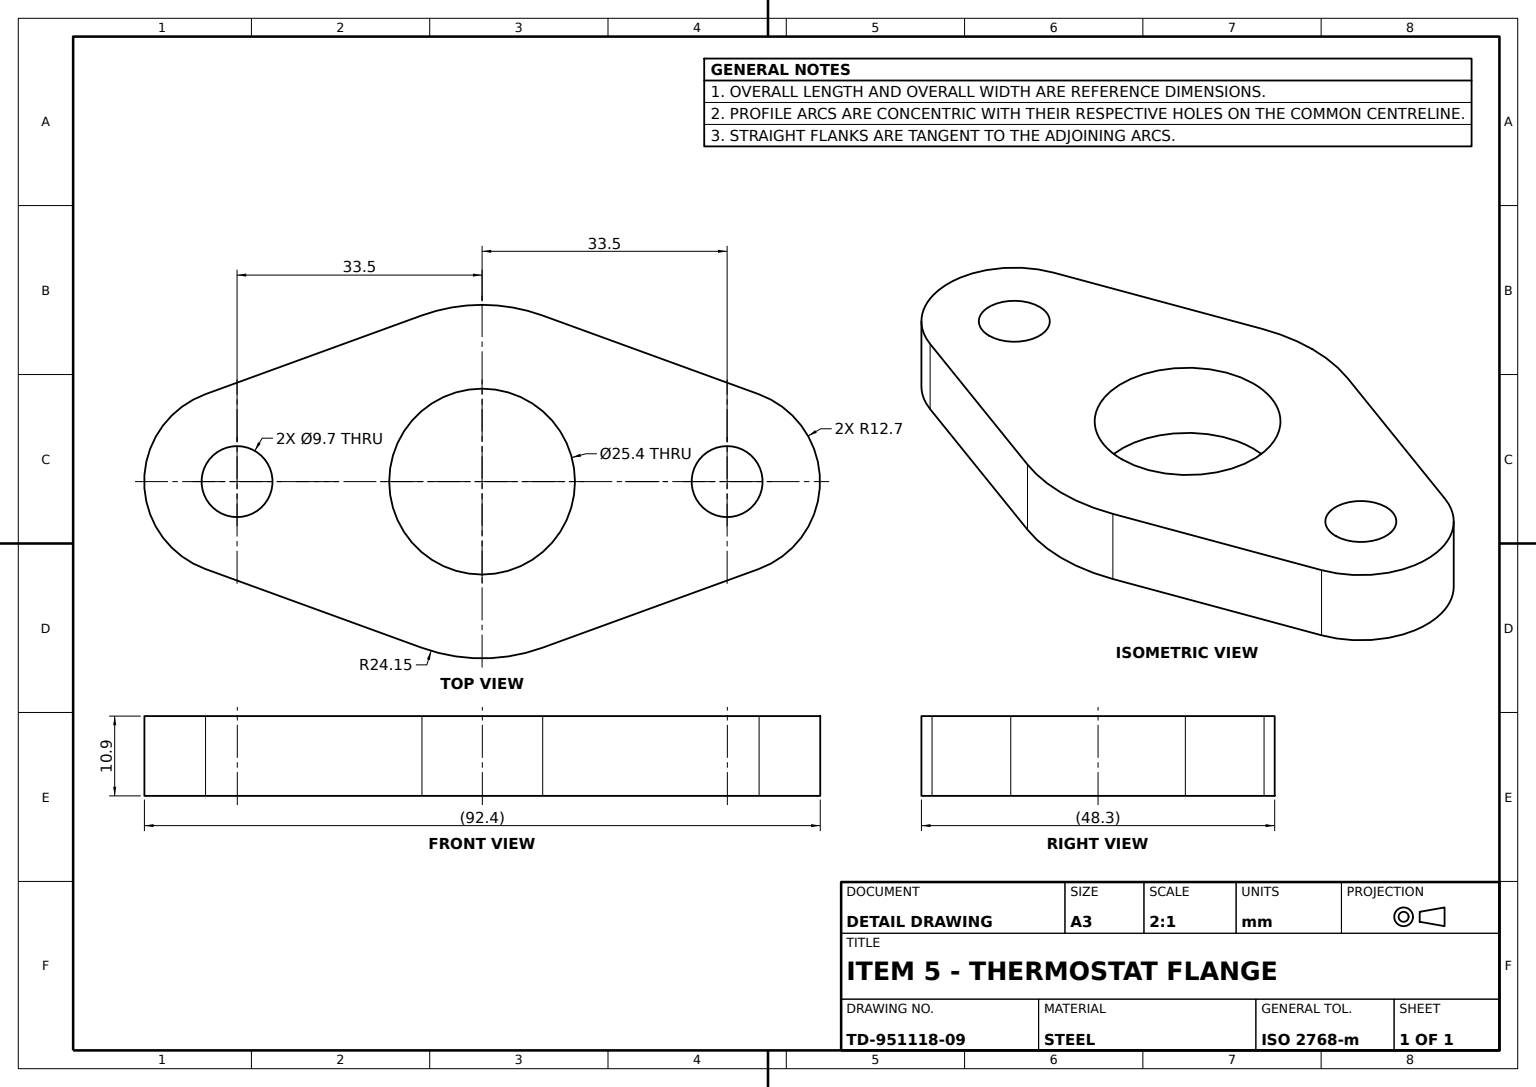
ISO-10303-21;
HEADER;
FILE_DESCRIPTION((''),'2;1');
FILE_NAME('','',(''),(''),'','','');
FILE_SCHEMA(('AUTOMOTIVE_DESIGN'));
ENDSEC;
DATA;
#1=APPLICATION_CONTEXT('');
#2=PRODUCT_CONTEXT('',#1,'mechanical');
#3=PRODUCT('','','',(#2));
#4=PRODUCT_DEFINITION_FORMATION('','',#3);
#5=PRODUCT_DEFINITION_CONTEXT('',#1,'design');
#6=PRODUCT_DEFINITION('','',#4,#5);
#7=PRODUCT_DEFINITION_SHAPE('','',#6);
#8=(LENGTH_UNIT()NAMED_UNIT(*)SI_UNIT(.MILLI.,.METRE.));
#9=(NAMED_UNIT(*)PLANE_ANGLE_UNIT()SI_UNIT($,.RADIAN.));
#10=(NAMED_UNIT(*)SI_UNIT($,.STERADIAN.)SOLID_ANGLE_UNIT());
#11=UNCERTAINTY_MEASURE_WITH_UNIT(LENGTH_MEASURE(1.E-05),#8,'distance_accuracy_value','');
#12=(GEOMETRIC_REPRESENTATION_CONTEXT(3)GLOBAL_UNCERTAINTY_ASSIGNED_CONTEXT((#11))GLOBAL_UNIT_ASSIGNED_CONTEXT((#8,#9,#10))REPRESENTATION_CONTEXT('',''));
#13=CARTESIAN_POINT('',(-12.7,0.,10.9));
#14=VERTEX_POINT('',#13);
#15=CARTESIAN_POINT('',(12.7,0.,10.9));
#16=VERTEX_POINT('',#15);
#17=CARTESIAN_POINT('',(0.,0.,10.9));
#18=DIRECTION('',(0.,0.,1.));
#19=DIRECTION('',(1.,0.,0.));
#20=AXIS2_PLACEMENT_3D('',#17,#18,#19);
#21=CIRCLE('',#20,12.7);
#22=EDGE_CURVE('',#14,#16,#21,.T.);
#23=ORIENTED_EDGE('',*,*,#22,.T.);
#24=CARTESIAN_POINT('',(12.7,0.,0.));
#25=VERTEX_POINT('',#24);
#26=CARTESIAN_POINT('',(12.7,0.,-39.));
#27=VECTOR('',#18,1000.);
#28=LINE('',#26,#27);
#29=EDGE_CURVE('',#25,#16,#28,.T.);
#30=ORIENTED_EDGE('',*,*,#29,.F.);
#31=CARTESIAN_POINT('',(-12.7,0.,0.));
#32=VERTEX_POINT('',#31);
#33=CARTESIAN_POINT('',(0.,0.,0.));
#34=DIRECTION('',(0.,0.,-1.));
#35=DIRECTION('',(-1.,0.,0.));
#36=AXIS2_PLACEMENT_3D('',#33,#34,#35);
#37=CIRCLE('',#36,12.7);
#38=EDGE_CURVE('',#25,#32,#37,.T.);
#39=ORIENTED_EDGE('',*,*,#38,.T.);
#40=CARTESIAN_POINT('',(-12.7,0.,-39.));
#41=LINE('',#40,#27);
#42=EDGE_CURVE('',#32,#14,#41,.T.);
#43=ORIENTED_EDGE('',*,*,#42,.T.);
#44=EDGE_LOOP('',(#23,#30,#39,#43));
#45=FACE_OUTER_BOUND('',#44,.T.);
#46=CARTESIAN_POINT('',(0.,0.,-39.));
#47=AXIS2_PLACEMENT_3D('',#46,#18,#19);
#48=CYLINDRICAL_SURFACE('',#47,12.7);
#49=ADVANCED_FACE('',(#45),#48,.F.);
#50=CARTESIAN_POINT('',(22.69559,8.254254,10.9));
#51=VERTEX_POINT('',#50);
#52=CARTESIAN_POINT('',(11.935155,37.840746,10.9));
#53=VERTEX_POINT('',#52);
#54=DIRECTION('',(-0.341791045,0.939775974,0.));
#55=VECTOR('',#54,1000.);
#56=LINE('',#52,#55);
#57=EDGE_CURVE('',#51,#53,#56,.T.);
#58=ORIENTED_EDGE('',*,*,#57,.T.);
#59=CARTESIAN_POINT('',(-11.935155,37.840746,10.9));
#60=VERTEX_POINT('',#59);
#61=CARTESIAN_POINT('',(0.,33.5,10.9));
#62=AXIS2_PLACEMENT_3D('',#61,#18,#19);
#63=CIRCLE('',#62,12.7);
#64=EDGE_CURVE('',#53,#60,#63,.T.);
#65=ORIENTED_EDGE('',*,*,#64,.T.);
#66=CARTESIAN_POINT('',(-22.69559,8.254254,10.9));
#67=VERTEX_POINT('',#66);
#68=DIRECTION('',(-0.341791045,-0.939775974,0.));
#69=VECTOR('',#68,1000.);
#70=LINE('',#59,#69);
#71=EDGE_CURVE('',#60,#67,#70,.T.);
#72=ORIENTED_EDGE('',*,*,#71,.T.);
#73=CARTESIAN_POINT('',(-24.15,0.,10.9));
#74=VERTEX_POINT('',#73);
#75=CIRCLE('',#20,24.15);
#76=EDGE_CURVE('',#67,#74,#75,.T.);
#77=ORIENTED_EDGE('',*,*,#76,.T.);
#78=CARTESIAN_POINT('',(-22.69559,-8.254254,10.9));
#79=VERTEX_POINT('',#78);
#80=EDGE_CURVE('',#74,#79,#75,.T.);
#81=ORIENTED_EDGE('',*,*,#80,.T.);
#82=CARTESIAN_POINT('',(-11.935155,-37.840746,10.9));
#83=VERTEX_POINT('',#82);
#84=DIRECTION('',(0.341791045,-0.939775974,0.));
#85=VECTOR('',#84,1000.);
#86=LINE('',#82,#85);
#87=EDGE_CURVE('',#79,#83,#86,.T.);
#88=ORIENTED_EDGE('',*,*,#87,.T.);
#89=CARTESIAN_POINT('',(11.935155,-37.840746,10.9));
#90=VERTEX_POINT('',#89);
#91=CARTESIAN_POINT('',(0.,-33.5,10.9));
#92=AXIS2_PLACEMENT_3D('',#91,#18,#35);
#93=CIRCLE('',#92,12.7);
#94=EDGE_CURVE('',#83,#90,#93,.T.);
#95=ORIENTED_EDGE('',*,*,#94,.T.);
#96=CARTESIAN_POINT('',(22.69559,-8.254254,10.9));
#97=VERTEX_POINT('',#96);
#98=DIRECTION('',(0.341791045,0.939775974,0.));
#99=VECTOR('',#98,1000.);
#100=LINE('',#89,#99);
#101=EDGE_CURVE('',#90,#97,#100,.T.);
#102=ORIENTED_EDGE('',*,*,#101,.T.);
#103=EDGE_CURVE('',#97,#51,#75,.T.);
#104=ORIENTED_EDGE('',*,*,#103,.T.);
#105=EDGE_LOOP('',(#58,#65,#72,#77,#81,#88,#95,#102,#104));
#106=FACE_OUTER_BOUND('',#105,.T.);
#107=CARTESIAN_POINT('',(4.85,-33.5,10.9));
#108=VERTEX_POINT('',#107);
#109=CARTESIAN_POINT('',(-4.85,-33.5,10.9));
#110=VERTEX_POINT('',#109);
#111=AXIS2_PLACEMENT_3D('',#91,#18,#19);
#112=CIRCLE('',#111,4.85);
#113=EDGE_CURVE('',#108,#110,#112,.T.);
#114=ORIENTED_EDGE('',*,*,#113,.F.);
#115=EDGE_CURVE('',#110,#108,#112,.T.);
#116=ORIENTED_EDGE('',*,*,#115,.F.);
#117=EDGE_LOOP('',(#114,#116));
#118=FACE_BOUND('',#117,.T.);
#119=CARTESIAN_POINT('',(-4.85,33.5,10.9));
#120=VERTEX_POINT('',#119);
#121=CARTESIAN_POINT('',(4.85,33.5,10.9));
#122=VERTEX_POINT('',#121);
#123=CIRCLE('',#62,4.85);
#124=EDGE_CURVE('',#120,#122,#123,.T.);
#125=ORIENTED_EDGE('',*,*,#124,.F.);
#126=EDGE_CURVE('',#122,#120,#123,.T.);
#127=ORIENTED_EDGE('',*,*,#126,.F.);
#128=EDGE_LOOP('',(#125,#127));
#129=FACE_BOUND('',#128,.T.);
#130=ORIENTED_EDGE('',*,*,#22,.F.);
#131=EDGE_CURVE('',#16,#14,#21,.T.);
#132=ORIENTED_EDGE('',*,*,#131,.F.);
#133=EDGE_LOOP('',(#130,#132));
#134=FACE_BOUND('',#133,.T.);
#135=AXIS2_PLACEMENT_3D('',#91,#34,#35);
#136=PLANE('',#135);
#137=ADVANCED_FACE('',(#106,#118,#129,#134),#136,.F.);
#138=CARTESIAN_POINT('',(-4.85,-33.5,0.));
#139=VERTEX_POINT('',#138);
#140=CARTESIAN_POINT('',(4.85,-33.5,0.));
#141=VERTEX_POINT('',#140);
#142=CARTESIAN_POINT('',(0.,-33.5,0.));
#143=AXIS2_PLACEMENT_3D('',#142,#34,#35);
#144=CIRCLE('',#143,4.85);
#145=EDGE_CURVE('',#139,#141,#144,.T.);
#146=ORIENTED_EDGE('',*,*,#145,.T.);
#147=CARTESIAN_POINT('',(4.85,-33.5,-39.));
#148=LINE('',#147,#27);
#149=EDGE_CURVE('',#141,#108,#148,.T.);
#150=ORIENTED_EDGE('',*,*,#149,.T.);
#151=ORIENTED_EDGE('',*,*,#113,.T.);
#152=CARTESIAN_POINT('',(-4.85,-33.5,-39.));
#153=LINE('',#152,#27);
#154=EDGE_CURVE('',#139,#110,#153,.T.);
#155=ORIENTED_EDGE('',*,*,#154,.F.);
#156=EDGE_LOOP('',(#146,#150,#151,#155));
#157=FACE_OUTER_BOUND('',#156,.T.);
#158=CARTESIAN_POINT('',(0.,-33.5,-39.));
#159=AXIS2_PLACEMENT_3D('',#158,#18,#19);
#160=CYLINDRICAL_SURFACE('',#159,4.85);
#161=ADVANCED_FACE('',(#157),#160,.F.);
#162=ORIENTED_EDGE('',*,*,#115,.T.);
#163=ORIENTED_EDGE('',*,*,#149,.F.);
#164=EDGE_CURVE('',#141,#139,#144,.T.);
#165=ORIENTED_EDGE('',*,*,#164,.T.);
#166=ORIENTED_EDGE('',*,*,#154,.T.);
#167=EDGE_LOOP('',(#162,#163,#165,#166));
#168=FACE_OUTER_BOUND('',#167,.T.);
#169=ADVANCED_FACE('',(#168),#160,.F.);
#170=CARTESIAN_POINT('',(4.85,33.5,0.));
#171=VERTEX_POINT('',#170);
#172=CARTESIAN_POINT('',(4.85,33.5,-39.));
#173=LINE('',#172,#27);
#174=EDGE_CURVE('',#171,#122,#173,.T.);
#175=ORIENTED_EDGE('',*,*,#174,.F.);
#176=CARTESIAN_POINT('',(-4.85,33.5,0.));
#177=VERTEX_POINT('',#176);
#178=CARTESIAN_POINT('',(0.,33.5,0.));
#179=AXIS2_PLACEMENT_3D('',#178,#34,#35);
#180=CIRCLE('',#179,4.85);
#181=EDGE_CURVE('',#171,#177,#180,.T.);
#182=ORIENTED_EDGE('',*,*,#181,.T.);
#183=CARTESIAN_POINT('',(-4.85,33.5,-39.));
#184=LINE('',#183,#27);
#185=EDGE_CURVE('',#177,#120,#184,.T.);
#186=ORIENTED_EDGE('',*,*,#185,.T.);
#187=ORIENTED_EDGE('',*,*,#124,.T.);
#188=EDGE_LOOP('',(#175,#182,#186,#187));
#189=FACE_OUTER_BOUND('',#188,.T.);
#190=CARTESIAN_POINT('',(0.,33.5,-39.));
#191=AXIS2_PLACEMENT_3D('',#190,#18,#19);
#192=CYLINDRICAL_SURFACE('',#191,4.85);
#193=ADVANCED_FACE('',(#189),#192,.F.);
#194=CARTESIAN_POINT('',(-24.15,0.,0.));
#195=VERTEX_POINT('',#194);
#196=CARTESIAN_POINT('',(-22.69559,-8.254254,0.));
#197=VERTEX_POINT('',#196);
#198=AXIS2_PLACEMENT_3D('',#33,#18,#19);
#199=CIRCLE('',#198,24.15);
#200=EDGE_CURVE('',#195,#197,#199,.T.);
#201=ORIENTED_EDGE('',*,*,#200,.T.);
#202=VECTOR('',#34,1000.);
#203=LINE('',#78,#202);
#204=EDGE_CURVE('',#79,#197,#203,.T.);
#205=ORIENTED_EDGE('',*,*,#204,.F.);
#206=ORIENTED_EDGE('',*,*,#80,.F.);
#207=LINE('',#73,#202);
#208=EDGE_CURVE('',#74,#195,#207,.T.);
#209=ORIENTED_EDGE('',*,*,#208,.T.);
#210=EDGE_LOOP('',(#201,#205,#206,#209));
#211=FACE_OUTER_BOUND('',#210,.T.);
#212=AXIS2_PLACEMENT_3D('',#17,#34,#35);
#213=CYLINDRICAL_SURFACE('',#212,24.15);
#214=ADVANCED_FACE('',(#211),#213,.T.);
#215=ORIENTED_EDGE('',*,*,#64,.F.);
#216=CARTESIAN_POINT('',(11.935155,37.840746,0.));
#217=VERTEX_POINT('',#216);
#218=LINE('',#52,#202);
#219=EDGE_CURVE('',#53,#217,#218,.T.);
#220=ORIENTED_EDGE('',*,*,#219,.T.);
#221=CARTESIAN_POINT('',(-11.935155,37.840746,0.));
#222=VERTEX_POINT('',#221);
#223=AXIS2_PLACEMENT_3D('',#178,#18,#19);
#224=CIRCLE('',#223,12.7);
#225=EDGE_CURVE('',#217,#222,#224,.T.);
#226=ORIENTED_EDGE('',*,*,#225,.T.);
#227=LINE('',#59,#202);
#228=EDGE_CURVE('',#60,#222,#227,.T.);
#229=ORIENTED_EDGE('',*,*,#228,.F.);
#230=EDGE_LOOP('',(#215,#220,#226,#229));
#231=FACE_OUTER_BOUND('',#230,.T.);
#232=AXIS2_PLACEMENT_3D('',#61,#34,#35);
#233=CYLINDRICAL_SURFACE('',#232,12.7);
#234=ADVANCED_FACE('',(#231),#233,.T.);
#235=CARTESIAN_POINT('',(-11.935155,-37.840746,0.));
#236=VERTEX_POINT('',#235);
#237=CARTESIAN_POINT('',(11.935155,-37.840746,0.));
#238=VERTEX_POINT('',#237);
#239=AXIS2_PLACEMENT_3D('',#142,#18,#35);
#240=CIRCLE('',#239,12.7);
#241=EDGE_CURVE('',#236,#238,#240,.T.);
#242=ORIENTED_EDGE('',*,*,#241,.T.);
#243=LINE('',#89,#202);
#244=EDGE_CURVE('',#90,#238,#243,.T.);
#245=ORIENTED_EDGE('',*,*,#244,.F.);
#246=ORIENTED_EDGE('',*,*,#94,.F.);
#247=LINE('',#82,#202);
#248=EDGE_CURVE('',#83,#236,#247,.T.);
#249=ORIENTED_EDGE('',*,*,#248,.T.);
#250=EDGE_LOOP('',(#242,#245,#246,#249));
#251=FACE_OUTER_BOUND('',#250,.T.);
#252=CYLINDRICAL_SURFACE('',#135,12.7);
#253=ADVANCED_FACE('',(#251),#252,.T.);
#254=ORIENTED_EDGE('',*,*,#87,.F.);
#255=ORIENTED_EDGE('',*,*,#204,.T.);
#256=LINE('',#235,#85);
#257=EDGE_CURVE('',#197,#236,#256,.T.);
#258=ORIENTED_EDGE('',*,*,#257,.T.);
#259=ORIENTED_EDGE('',*,*,#248,.F.);
#260=EDGE_LOOP('',(#254,#255,#258,#259));
#261=FACE_OUTER_BOUND('',#260,.T.);
#262=DIRECTION('',(0.939775974,0.341791045,0.));
#263=AXIS2_PLACEMENT_3D('',#82,#262,#54);
#264=PLANE('',#263);
#265=ADVANCED_FACE('',(#261),#264,.F.);
#266=ORIENTED_EDGE('',*,*,#244,.T.);
#267=CARTESIAN_POINT('',(22.69559,-8.254254,0.));
#268=VERTEX_POINT('',#267);
#269=LINE('',#237,#99);
#270=EDGE_CURVE('',#238,#268,#269,.T.);
#271=ORIENTED_EDGE('',*,*,#270,.T.);
#272=LINE('',#96,#202);
#273=EDGE_CURVE('',#97,#268,#272,.T.);
#274=ORIENTED_EDGE('',*,*,#273,.F.);
#275=ORIENTED_EDGE('',*,*,#101,.F.);
#276=EDGE_LOOP('',(#266,#271,#274,#275));
#277=FACE_OUTER_BOUND('',#276,.T.);
#278=DIRECTION('',(-0.939775974,0.341791045,0.));
#279=AXIS2_PLACEMENT_3D('',#89,#278,#68);
#280=PLANE('',#279);
#281=ADVANCED_FACE('',(#277),#280,.F.);
#282=CARTESIAN_POINT('',(22.69559,8.254254,0.));
#283=VERTEX_POINT('',#282);
#284=EDGE_CURVE('',#268,#283,#199,.T.);
#285=ORIENTED_EDGE('',*,*,#284,.T.);
#286=LINE('',#50,#202);
#287=EDGE_CURVE('',#51,#283,#286,.T.);
#288=ORIENTED_EDGE('',*,*,#287,.F.);
#289=ORIENTED_EDGE('',*,*,#103,.F.);
#290=ORIENTED_EDGE('',*,*,#273,.T.);
#291=EDGE_LOOP('',(#285,#288,#289,#290));
#292=FACE_OUTER_BOUND('',#291,.T.);
#293=ADVANCED_FACE('',(#292),#213,.T.);
#294=ORIENTED_EDGE('',*,*,#208,.F.);
#295=ORIENTED_EDGE('',*,*,#76,.F.);
#296=CARTESIAN_POINT('',(-22.69559,8.254254,0.));
#297=VERTEX_POINT('',#296);
#298=LINE('',#66,#202);
#299=EDGE_CURVE('',#67,#297,#298,.T.);
#300=ORIENTED_EDGE('',*,*,#299,.T.);
#301=EDGE_CURVE('',#297,#195,#199,.T.);
#302=ORIENTED_EDGE('',*,*,#301,.T.);
#303=EDGE_LOOP('',(#294,#295,#300,#302));
#304=FACE_OUTER_BOUND('',#303,.T.);
#305=ADVANCED_FACE('',(#304),#213,.T.);
#306=ORIENTED_EDGE('',*,*,#131,.T.);
#307=ORIENTED_EDGE('',*,*,#42,.F.);
#308=EDGE_CURVE('',#32,#25,#37,.T.);
#309=ORIENTED_EDGE('',*,*,#308,.T.);
#310=ORIENTED_EDGE('',*,*,#29,.T.);
#311=EDGE_LOOP('',(#306,#307,#309,#310));
#312=FACE_OUTER_BOUND('',#311,.T.);
#313=ADVANCED_FACE('',(#312),#48,.F.);
#314=ORIENTED_EDGE('',*,*,#71,.F.);
#315=ORIENTED_EDGE('',*,*,#228,.T.);
#316=LINE('',#221,#69);
#317=EDGE_CURVE('',#222,#297,#316,.T.);
#318=ORIENTED_EDGE('',*,*,#317,.T.);
#319=ORIENTED_EDGE('',*,*,#299,.F.);
#320=EDGE_LOOP('',(#314,#315,#318,#319));
#321=FACE_OUTER_BOUND('',#320,.T.);
#322=DIRECTION('',(0.939775974,-0.341791045,0.));
#323=AXIS2_PLACEMENT_3D('',#59,#322,#98);
#324=PLANE('',#323);
#325=ADVANCED_FACE('',(#321),#324,.F.);
#326=ORIENTED_EDGE('',*,*,#126,.T.);
#327=ORIENTED_EDGE('',*,*,#185,.F.);
#328=EDGE_CURVE('',#177,#171,#180,.T.);
#329=ORIENTED_EDGE('',*,*,#328,.T.);
#330=ORIENTED_EDGE('',*,*,#174,.T.);
#331=EDGE_LOOP('',(#326,#327,#329,#330));
#332=FACE_OUTER_BOUND('',#331,.T.);
#333=ADVANCED_FACE('',(#332),#192,.F.);
#334=ORIENTED_EDGE('',*,*,#38,.F.);
#335=ORIENTED_EDGE('',*,*,#308,.F.);
#336=EDGE_LOOP('',(#334,#335));
#337=FACE_BOUND('',#336,.T.);
#338=ORIENTED_EDGE('',*,*,#164,.F.);
#339=ORIENTED_EDGE('',*,*,#145,.F.);
#340=EDGE_LOOP('',(#338,#339));
#341=FACE_BOUND('',#340,.T.);
#342=ORIENTED_EDGE('',*,*,#181,.F.);
#343=ORIENTED_EDGE('',*,*,#328,.F.);
#344=EDGE_LOOP('',(#342,#343));
#345=FACE_BOUND('',#344,.T.);
#346=ORIENTED_EDGE('',*,*,#317,.F.);
#347=ORIENTED_EDGE('',*,*,#225,.F.);
#348=LINE('',#216,#55);
#349=EDGE_CURVE('',#283,#217,#348,.T.);
#350=ORIENTED_EDGE('',*,*,#349,.F.);
#351=ORIENTED_EDGE('',*,*,#284,.F.);
#352=ORIENTED_EDGE('',*,*,#270,.F.);
#353=ORIENTED_EDGE('',*,*,#241,.F.);
#354=ORIENTED_EDGE('',*,*,#257,.F.);
#355=ORIENTED_EDGE('',*,*,#200,.F.);
#356=ORIENTED_EDGE('',*,*,#301,.F.);
#357=EDGE_LOOP('',(#346,#347,#350,#351,#352,#353,#354,#355,#356));
#358=FACE_OUTER_BOUND('',#357,.T.);
#359=PLANE('',#143);
#360=ADVANCED_FACE('',(#337,#341,#345,#358),#359,.T.);
#361=ORIENTED_EDGE('',*,*,#219,.F.);
#362=ORIENTED_EDGE('',*,*,#57,.F.);
#363=ORIENTED_EDGE('',*,*,#287,.T.);
#364=ORIENTED_EDGE('',*,*,#349,.T.);
#365=EDGE_LOOP('',(#361,#362,#363,#364));
#366=FACE_OUTER_BOUND('',#365,.T.);
#367=DIRECTION('',(-0.939775974,-0.341791045,0.));
#368=AXIS2_PLACEMENT_3D('',#52,#367,#84);
#369=PLANE('',#368);
#370=ADVANCED_FACE('',(#366),#369,.F.);
#371=CLOSED_SHELL('',(#49,#137,#161,#169,#193,#214,#234,#253,#265,#281,#293,#305,#313,#325,#333,#360,#370));
#372=MANIFOLD_SOLID_BREP('',#371);
#373=ADVANCED_BREP_SHAPE_REPRESENTATION('',(#372),#12);
#374=SHAPE_DEFINITION_REPRESENTATION(#7,#373);
ENDSEC;
END-ISO-10303-21;
